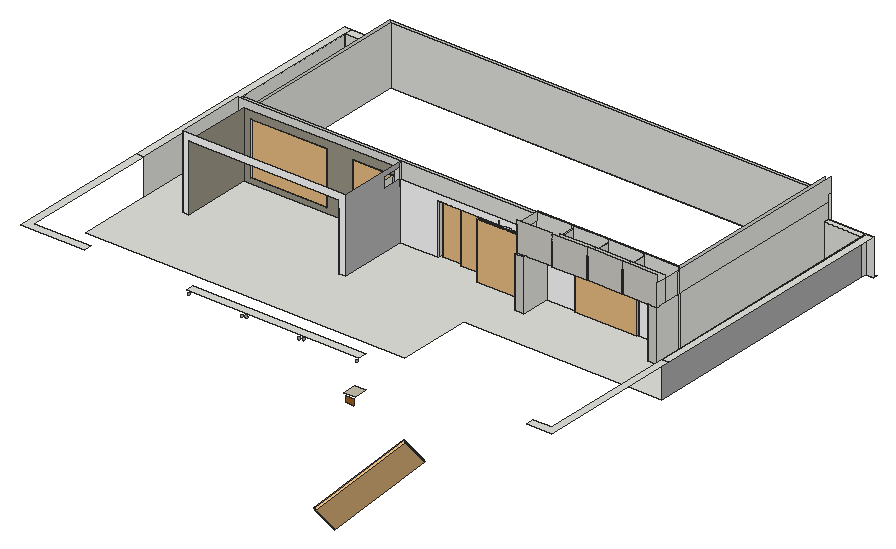
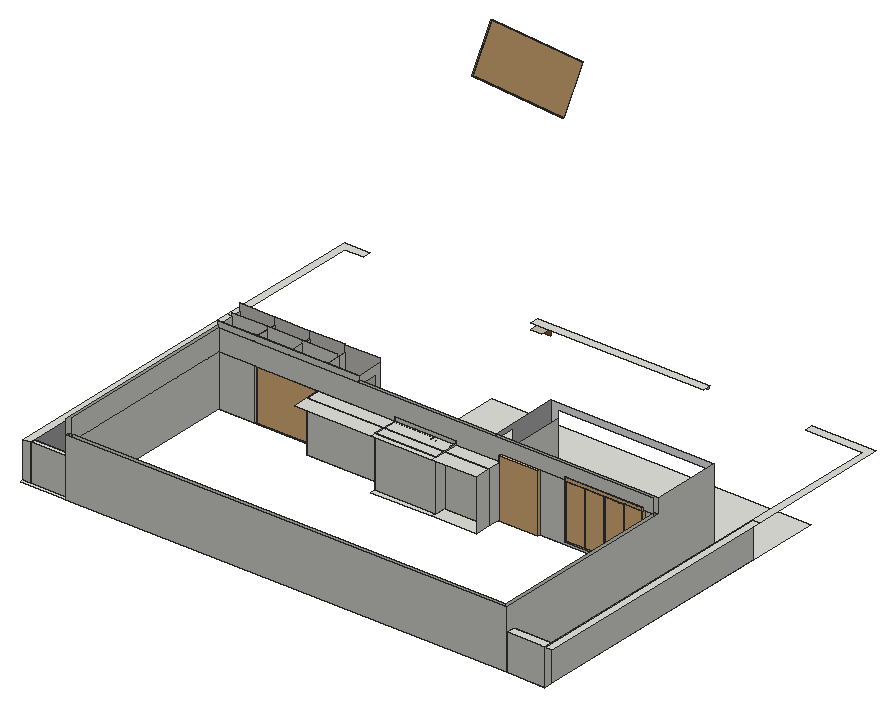
# SketchUp Ruby script. Lengths in inches.
U = 1.inch
M = Sketchup.active_model
def pt(a) = Geom::Point3d.new(a.map { |v| v * U })
def face(e, loops, mat)
  f = e.add_face(loops[0].map { |a| pt(a) })
  loops[1..].each { |l| e.add_face(l.map { |a| pt(a) }).erase! }
  f.material = f.back_material = mat if mat
  f
end
# faces: each face lists its corners as indices into pts; further lists are holes
def faces(e, pts, list, mat = nil) = list.each { |f| face(e, (f[0].is_a?(Array) ? f : [f]).map { |l| l.map { |i| pts[i] } }, mat) }
# xy, xz, yz: faces in a plane at the given z, y or x. An outline is a flat list of corners, or four numbers for a rectangle; further outlines are holes
def ring(l) = l.size == 4 ? [[l[0], l[1]], [l[2], l[1]], [l[2], l[3]], [l[0], l[3]]] : l.each_slice(2).to_a
def flat(e, list, mat, &to3) = list.each { |f| face(e, (f[0].is_a?(Array) ? f : [f]).map { |l| ring(l).map { |u, v| to3.(u, v) } }, mat) }
def xy(e, z, list, mat = nil) = flat(e, list, mat) { |x, y| [x, y, z] }
def xz(e, y, list, mat = nil) = flat(e, list, mat) { |x, z| [x, y, z] }
def yz(e, x, list, mat = nil) = flat(e, list, mat) { |y, z| [x, y, z] }
def lines(e, pts, list) = list.each { |a, b| e.add_line(pt(pts[a]), pt(pts[b])) }
# prism: a flat outline (further loops are holes) pulled along v
def prism(e, loops, v, mat = nil)
  f = face(e, loops, mat); d = Geom::Vector3d.new(v.map { |x| x * U })
  f.pushpull(f.normal.samedirection?(d) ? d.length : -d.length)
end
def box(e, o, s, mat = nil) = prism(e, [[o, [o[0] + s[0], o[1], o[2]], [o[0] + s[0], o[1] + s[1], o[2]], [o[0], o[1] + s[1], o[2]]]], [0, 0, s[2]], mat)
def at(x, y, z, deg = 0) = Geom::Transformation.translation(pt([x, y, z])) * Geom::Transformation.rotation(ORIGIN, Z_AXIS, deg.degrees)
def axes(o, x, y, z) = Geom::Transformation.new([*x, 0, *y, 0, *z, 0, *pt(o).to_a, 1])
def part(name) = M.definitions.add(name)
# library, detail: a bought-in or finely detailed component or shape, given as its bounding box
def library(name, o, s) = part(name).tap { |d| box(d.entities, o, s) }
def detail(e, o, s) = box(e.add_group.entities, o, s)
def put(e, d, t, mat = nil) = e.add_instance(d, t).tap { |i| i.material = mat if mat }
def group(e, t, mat = nil) = e.add_group.tap { |g| g.transformation = t; g.material = mat if mat }.entities
root = M.entities
M.materials.add("Material~3").color = [123, 113, 102]
M.materials.add("[0128_White]").color = [255, 255, 255]
M.materials.add("[0129_WhiteSmoke]").color = [178, 178, 178]
M.materials.add("[0132_LightGray]").color = [169, 169, 169]
M.materials.add("[Concrete Tile]").color = [155, 150, 134]
M.materials.add("[Terrazzo Tile Light]").color = [209, 207, 200]
M.materials.add("[Tile Canvas]").color = [199, 192, 173]
M.materials.add("[Wood Square Tile 02]").color = [160, 95, 34]
c1 = library("3DGeom~4_Defintion",[362.52,-15.59,12.6],[288.85,70.11,1000])
c2 = library("3 door",[0,0,0],[74.8,3.9375,43.31])
c3 = library("door (1)",[38.93,25.48,0],[40,9.94,82.68])
c4 = library("JALI+PATTERN-03",[8.875,53.125,6.4375],[84,1,53.5])
c5 = library("Group\#167",[0,0,0],[77.52,5,145.33])
xy(root,5.1875,[[[2048.43,611.53,2576.35,611.53,2576.35,732.28,2904.07,732.28,2904.07,1146.63,2840.8125,1146.63,2840.8125,851.0625,2671.4,851.0625,2671.4,845.35,2623.94,845.35,2623.94,798.41,2608.61,798.41,2608.61,845.35,2544.33,845.35,2544.33,874.25,2444.05,874.25,2444.05,845.35,2381.36,845.35,2381.36,732.28,2370.42,732.28,2370.42,851.0625,2305.05,851.0625,2305.05,845.35,2123,845.35,2123,732.28,2112.0625,732.28,2112.0625,1146.63,2048.43,1146.63],[2825.48,801.78,2840.8125,845.35]],[2112.0625,732.28,2112.0625,1160.85,2916.0625,1160.85,2916.0625,1155.13,2117.78,1155.13,2117.78,851.0625,2305.05,851.0625,2305.05,845.35,2123,845.35,2123,732.28],[2370.42,732.28,2370.42,846.1,2444.05,846.1,2444.05,845.35,2381.36,845.35,2381.36,732.28],[2608.61,798.41,2608.61,845.35,2544.33,845.35,2544.33,846.1,2671.4,846.1,2671.4,845.35,2623.94,845.35,2623.94,798.41],[2825.48,801.78,2840.8125,845.35],
  [2370.42,846.1,2444.05,874.25],[2544.33,846.1,2671.4,874.25],[2835.1,851.0625,2840.8125,1155.13],[2370.42,874.25,2444.05,900.375],[2444.05,874.25,2544.33,892.35],
  [2444.05,892.35,2544.33,900.375],[2048.43,1146.63,2112.0625,1160.85],[2840.8125,1146.63,2904.07,1155.13]])
xy(root,13.84,[[2134.72,845.35,2259.6,851.0625]])
xy(root,32.74,[[2602.58,453.42,2621.02,475.99]],"[Tile Canvas]")
xy(root,65.1875,[[2036.8125,491.47,2142.71,491.47,2142.71,505.1,2048.43,505.1,2048.43,732.28,2036.8125,732.28],[2311.71,491.47,2596.56,505.1],[2873.37,491.47,2916.0625,491.47,2916.0625,732.28,2904.07,732.28,2904.07,505.1,2873.37,505.1],[2036.8125,732.28,2048.43,1160.85],[2904.07,732.28,2916.0625,1155.13],
  [2048.43,1146.63,2112.0625,1160.85],[2840.8125,1146.63,2904.07,1155.13]])
xy(root,89.42,[[2608.61,798.41,2623.94,801.78],[2623.94,801.78,2666.66,814.22],[2667.6,801.78,2671.4,817.6],[2671.4,801.78,2724.71,817.6],[2725.77,801.78,2776.01,817.6],
  [2776.01,801.78,2782.76,817.6],[2784.08,801.78,2825.48,817.6],[2825.48,801.78,2840.8125,817.6],[2623.94,814.22,2666.66,844.47],[2667.6,817.6,2671.4,844.47],
  [2671.4,817.6,2724.71,844.47],[2725.77,817.6,2776.01,844.47],[2776.01,817.6,2782.76,844.47],[2784.08,817.6,2825.48,844.47],[2825.48,817.6,2840.8125,844.47],
  [2608.61,844.47,2623.94,845.35],[2623.94,844.47,2671.4,845.35],[2671.4,844.47,2776.01,845.35],[2776.01,844.47,2825.48,845.35],[2825.48,844.47,2840.8125,845.35],
  [2444.05,845.35,2544.33,846.1],[2544.33,845.35,2608.61,846.1],[2608.61,845.35,2671.4,846.1],[2671.4,845.35,2776.01,846.1],[2776.01,845.35,2840.8125,846.1],
  [2370.42,846.1,2444.05,851.0625],[2544.33,846.1,2671.4,851.0625],[2671.4,846.1,2776.01,851.0625],[2776.01,846.1,2840.8125,851.0625],[2370.42,851.0625,2444.05,874.25],
  [2444.05,851.0625,2544.33,874.25],[2544.33,851.0625,2671.4,874.25],[2835.1,851.0625,2840.8125,1155.13],[2370.42,874.25,2444.05,900.375],[2444.05,874.25,2544.33,892.35],
  [2544.33,874.25,2671.4,900.375],[2444.05,892.35,2544.33,900.375]])
xz(root,453.42,[[2604.93,19.53,2619.05,29.34]],"[Wood Square Tile 02]")
xz(root,491.47,[[2402.92,57.74,2403.41,57.8,2403.86,57.99,2404.25,58.29,2404.55,58.68,2404.73,59.13,2404.8,59.61,2404.73,60.1,2404.55,60.55,2404.25,60.94,2403.86,61.24,2403.41,61.43,2402.92,61.49,2402.4375,61.43,2401.99,61.24,2401.6,60.94,2401.3,60.55,2401.11,60.1,2401.05,59.61,2401.11,59.13,2401.3,58.68,2401.6,58.29,2401.99,57.99,2402.4375,57.8],[2497.875,57.74,2498.36,57.8,2498.8125,57.99,2499.2,58.29,2499.5,58.68,2499.69,59.13,2499.75,59.61,2499.69,60.1,2499.5,60.55,2499.2,60.94,2498.8125,61.24,2498.36,61.43,2497.875,61.49,2497.39,61.43,2496.9375,61.24,2496.55,60.94,2496.25,60.55,2496.0625,60.1,2496,59.61,2496.0625,59.13,2496.25,58.68,2496.55,58.29,2496.9375,57.99,2497.39,57.8],[2592.82,57.74,2593.31,57.8,2593.76,57.99,2594.15,58.29,2594.45,58.68,2594.64,59.13,2594.7,59.61,2594.64,60.1,2594.45,60.55,2594.15,60.94,2593.76,61.24,2593.31,61.43,2592.82,61.49,2592.34,61.43,2591.89,61.24,2591.5,60.94,2591.2,60.55,2591.01,60.1,2590.95,59.61,2591.01,59.13,2591.2,58.68,2591.5,58.29,2591.89,57.99,2592.34,57.8],[2315.19,59.21,2315.68,59.22,2316.15,59.36,2316.57,59.61,2316.9,59.97,2317.14,60.4,2317.25,60.875,2317.24,61.36,2317.1,61.83,2316.85,62.25,2316.49,62.59,2316.07,62.82,2315.59,62.9375,2315.1,62.93,2314.63,62.79,2314.21,62.53,2313.875,62.18,2313.64,61.75,2313.53,61.27,2313.54,60.78,2313.68,60.32,2313.93,59.9,2314.28,59.56,2314.71,59.33],[2410.14,59.21,2410.63,59.22,2411.1,59.36,2411.52,59.61,2411.86,59.97,2412.09,60.4,2412.2,60.875,2412.19,61.36,2412.05,61.83,2411.8,62.25,2411.45,62.59,2411.02,62.82,2410.54,62.9375,2410.05,62.93,2409.58,62.79,2409.16,62.53,2408.83,62.18,2408.59,61.75,2408.48,61.27,2408.49,60.78,2408.625,60.32,2408.88,59.9,2409.24,59.56,2409.67,59.33],
  [2505.09,59.21,2505.58,59.22,2506.05,59.36,2506.47,59.61,2506.81,59.97,2507.04,60.4,2507.16,60.875,2507.14,61.36,2507.01,61.83,2506.75,62.25,2506.4,62.59,2505.97,62.82,2505.49,62.9375,2505,62.93,2504.53,62.79,2504.11,62.53,2503.78,62.18,2503.54,61.75,2503.43,61.27,2503.4375,60.78,2503.58,60.32,2503.83,59.9,2504.1875,59.56,2504.62,59.33]],"[0132_LightGray]")
xz(root,732.28,[[2112.0625,5.1875,2123,5.1875,2123,114.25,2370.42,114.25,2370.42,5.1875,2381.36,5.1875,2381.36,125.1875,2112.0625,125.1875]],"[0128_White]")
xz(root,798.41,[[2608.61,5.1875,2623.94,89.42]],"[Terrazzo Tile Light]")
xz(root,801.78,[[2825.48,5.1875,2840.8125,89.42],[[2608.61,89.42,2666.66,138.0625],[2612.5,131.88,2612.21,131.92,2611.93,132.03,2611.7,132.21,2611.52,132.44,2611.41,132.71,2611.37,133,2611.41,133.29,2611.52,133.57,2611.7,133.8,2611.93,133.98,2612.21,134.09,2612.5,134.13,2612.79,134.09,2613.06,133.98,2613.29,133.8,2613.47,133.57,2613.58,133.29,2613.62,133,2613.58,132.71,2613.47,132.44,2613.29,132.21,2613.06,132.03,2612.79,131.92],[2663.62,131.88,2663.33,131.92,2663.06,132.03,2662.83,132.21,2662.65,132.44,2662.53,132.71,2662.5,133,2662.53,133.29,2662.65,133.57,2662.83,133.8,2663.06,133.98,2663.33,134.09,2663.62,134.13,2663.91,134.09,2664.18,133.98,2664.42,133.8,2664.6,133.57,2664.71,133.29,2664.75,133,2664.71,132.71,2664.6,132.44,2664.42,132.21,2664.18,132.03,2663.91,131.92],[2663.62,91.63,2663.33,91.67,2663.06,91.78,2662.83,91.96,2662.65,92.19,2662.53,92.46,2662.5,92.75,2662.53,93.04,2662.65,93.32,2662.83,93.55,2663.06,93.73,2663.33,93.84,2663.62,93.88,2663.91,93.84,2664.18,93.73,2664.42,93.55,2664.6,93.32,2664.71,93.04,2664.75,92.75,2664.71,92.46,2664.6,92.19,2664.42,91.96,2664.18,91.78,2663.91,91.67],[2611.43,91.63,2611.14,91.67,2610.87,91.78,2610.64,91.96,2610.46,92.19,2610.35,92.46,2610.31,92.75,2610.35,93.04,2610.46,93.32,2610.64,93.55,2610.87,93.73,2611.14,93.84,2611.43,93.88,2611.73,93.84,2612,93.73,2612.23,93.55,2612.41,93.32,2612.52,93.04,2612.56,92.75,2612.52,92.46,2612.41,92.19,2612.23,91.96,2612,91.78,2611.73,91.67]],[[2667.6,89.42,2724.71,138.0625],[2671.48,131.88,2671.19,131.92,2670.92,132.03,2670.6875,132.21,2670.51,132.44,2670.4,132.71,2670.36,133,2670.4,133.29,2670.51,133.57,2670.6875,133.8,2670.92,133.98,2671.19,134.09,2671.48,134.13,2671.78,134.09,2672.05,133.98,2672.28,133.8,2672.46,133.57,2672.57,133.29,2672.61,133,2672.57,132.71,2672.46,132.44,2672.28,132.21,2672.05,132.03,2671.78,131.92],[2722.61,91.63,2722.32,91.67,2722.05,91.78,2721.8125,91.96,2721.64,92.19,2721.52,92.46,2721.48,92.75,2721.52,93.04,2721.64,93.32,2721.8125,93.55,2722.05,93.73,2722.32,93.84,2722.61,93.88,2722.9,93.84,2723.17,93.73,2723.41,93.55,2723.58,93.32,2723.7,93.04,2723.73,92.75,2723.7,92.46,2723.58,92.19,2723.41,91.96,2723.17,91.78,2722.9,91.67],[2670.42,91.63,2670.13,91.67,2669.86,91.78,2669.625,91.96,2669.45,92.19,2669.34,92.46,2669.3,92.75,2669.34,93.04,2669.45,93.32,2669.625,93.55,2669.86,93.73,2670.13,93.84,2670.42,93.88,2670.71,93.84,2670.98,93.73,2671.22,93.55,2671.4,93.32,2671.51,93.04,2671.55,92.75,2671.51,92.46,2671.4,92.19,2671.22,91.96,2670.98,91.78,2670.71,91.67],[2722.61,131.88,2722.32,131.92,2722.05,132.03,2721.8125,132.21,2721.64,132.44,2721.52,132.71,2721.48,133,2721.52,133.29,2721.64,133.57,2721.8125,133.8,2722.05,133.98,2722.32,134.09,2722.61,134.13,2722.9,134.09,2723.17,133.98,2723.41,133.8,2723.58,133.57,2723.7,133.29,2723.73,133,2723.7,132.71,2723.58,132.44,2723.41,132.21,2723.17,132.03,2722.9,131.92]],[[2725.77,89.42,2782.76,138.0625],[2780.79,131.88,2780.49,131.92,2780.22,132.03,2779.99,132.21,2779.8125,132.44,2779.7,132.71,2779.66,133,2779.7,133.29,2779.8125,133.57,2779.99,133.8,2780.22,133.98,2780.49,134.09,2780.79,134.13,2781.08,134.09,2781.35,133.98,2781.58,133.8,2781.76,133.57,2781.87,133.29,2781.91,133,2781.87,132.71,2781.76,132.44,2781.58,132.21,2781.35,132.03,2781.08,131.92],[2729.66,131.88,2729.37,131.92,2729.1,132.03,2728.86,132.21,2728.6875,132.44,2728.57,132.71,2728.54,133,2728.57,133.29,2728.6875,133.57,2728.86,133.8,2729.1,133.98,2729.37,134.09,2729.66,134.13,2729.95,134.09,2730.22,133.98,2730.46,133.8,2730.63,133.57,2730.75,133.29,2730.79,133,2730.75,132.71,2730.63,132.44,2730.46,132.21,2730.22,132.03,2729.95,131.92],[2780.79,91.63,2780.49,91.67,2780.22,91.78,2779.99,91.96,2779.8125,92.19,2779.7,92.46,2779.66,92.75,2779.7,93.04,2779.8125,93.32,2779.99,93.55,2780.22,93.73,2780.49,93.84,2780.79,93.88,2781.08,93.84,2781.35,93.73,2781.58,93.55,2781.76,93.32,2781.87,93.04,2781.91,92.75,2781.87,92.46,2781.76,92.19,2781.58,91.96,2781.35,91.78,2781.08,91.67],[2728.6,91.63,2728.31,91.67,2728.04,91.78,2727.8,91.96,2727.625,92.19,2727.51,92.46,2727.47,92.75,2727.51,93.04,2727.625,93.32,2727.8,93.55,2728.04,93.73,2728.31,93.84,2728.6,93.88,2728.89,93.84,2729.16,93.73,2729.39,93.55,2729.57,93.32,2729.68,93.04,2729.72,92.75,2729.68,92.46,2729.57,92.19,2729.39,91.96,2729.16,91.78,2728.89,91.67]],[[2784.08,89.42,2840.8125,138.0625],[2786.9,91.63,2786.61,91.67,2786.34,91.78,2786.1,91.96,2785.92,92.19,2785.8125,92.46,2785.77,92.75,2785.8125,93.04,2785.92,93.32,2786.1,93.55,2786.34,93.73,2786.61,93.84,2786.9,93.88,2787.19,93.84,2787.46,93.73,2787.69,93.55,2787.87,93.32,2787.99,93.04,2788.02,92.75,2787.99,92.46,2787.87,92.19,2787.69,91.96,2787.46,91.78,2787.19,91.67],[2787.96,131.88,2787.67,131.92,2787.4,132.03,2787.17,132.21,2786.99,132.44,2786.875,132.71,2786.84,133,2786.875,133.29,2786.99,133.57,2787.17,133.8,2787.4,133.98,2787.67,134.09,2787.96,134.13,2788.25,134.09,2788.52,133.98,2788.76,133.8,2788.94,133.57,2789.05,133.29,2789.09,133,2789.05,132.71,2788.94,132.44,2788.76,132.21,2788.52,132.03,2788.25,131.92],[2839.09,91.63,2838.8,91.67,2838.52,91.78,2838.29,91.96,2838.11,92.19,2838,92.46,2837.96,92.75,2838,93.04,2838.11,93.32,2838.29,93.55,2838.52,93.73,2838.8,93.84,2839.09,93.88,2839.38,93.84,2839.65,93.73,2839.88,93.55,2840.06,93.32,2840.17,93.04,2840.21,92.75,2840.17,92.46,2840.06,92.19,2839.88,91.96,2839.65,91.78,2839.38,91.67],[2839.09,131.88,2838.8,131.92,2838.52,132.03,2838.29,132.21,2838.11,132.44,2838,132.71,2837.96,133,2838,133.29,2838.11,133.57,2838.29,133.8,2838.52,133.98,2838.8,134.09,2839.09,134.13,2839.38,134.09,2839.65,133.98,2839.88,133.8,2840.06,133.57,2840.17,133.29,2840.21,133,2840.17,132.71,2840.06,132.44,2839.88,132.21,2839.65,132.03,2839.38,131.92]]],"[Terrazzo Tile Light]")
xz(root,817.6,[[2667.6,89.42,2724.71,131.1875],[2725.77,89.42,2782.76,131.1875],[2784.08,89.42,2840.8125,131.1875]])
xz(root,844.47,[[2608.61,89.42,2666.66,131.1875],[2666.66,89.42,2667.6,131.1875],[2667.6,89.42,2724.71,131.1875],[2724.71,89.42,2725.77,131.1875],[2725.77,89.42,2782.76,131.1875],
  [2782.76,89.42,2784.08,131.1875],[2784.08,89.42,2840.8125,131.1875]])
xz(root,845.35,[[2544.33,5.1875,2608.61,89.42],[2825.48,5.1875,2840.8125,89.42]])
xz(root,845.35,[[2381.36,5.1875,2444.05,5.1875,2444.05,89.42,2608.61,89.42,2608.61,99.26,2381.36,99.26],[2623.94,5.1875,2671.4,89.42],[2776.01,5.1875,2825.48,89.42]],"[0128_White]")
xz(root,845.35,[[[2123,5.1875,2305.05,5.1875,2305.05,101.375,2370.42,101.375,2370.42,114.25,2123,114.25],[2134.72,13.84,2259.6,101.78]]],"[Concrete Tile]")
xz(root,846.1,[[2370.42,5.1875,2444.05,89.42],[2544.33,5.1875,2671.4,89.42],[2370.42,89.42,2381.36,89.42,2381.36,125.1875,2112.0625,125.1875,2112.0625,101.375,2370.42,101.375],[2381.36,89.42,2381.36,125.1875,2608.61,125.1875,2608.61,89.42,2544.33,89.42,2544.33,95.79,2444.05,95.79,2444.05,89.42],[2444.05,89.42,2544.33,95.79],
  [2608.61,89.42,2840.8125,131.1875]])
xz(root,851.0625,[[2117.78,5.1875,2117.78,101.375,2134.72,101.375,2134.72,13.84,2259.6,13.84,2259.6,101.375,2305.05,101.375,2305.05,5.1875],[2776.01,5.1875,2835.1,89.42],[2835.1,5.1875,2840.8125,89.42],[2370.42,89.42,2370.42,101.375,2259.6,101.375,2259.6,101.78,2134.72,101.78,2134.72,101.375,2117.78,101.375,2117.78,125.1875,2835.1,125.1875,2835.1,89.42,2544.33,89.42,2544.33,95.79,2444.05,95.79,2444.05,89.42],[2444.05,89.42,2544.33,95.79]])
xz(root,874.25,[[2370.42,5.1875,2671.4,89.42]])
xz(root,892.35,[[2444.05,5.1875,2544.33,89.42]])
xz(root,1146.63,[[2048.43,5.1875,2112.0625,65.1875],[2840.8125,5.1875,2904.07,65.1875]])
xz(root,1155.13,[[2117.78,5.1875,2835.1,101.375],[2835.1,5.1875,2840.8125,89.42],[2840.8125,5.1875,2904.07,65.1875],[2904.07,5.1875,2916.0625,65.1875],[2835.1,89.42,2840.8125,101.375]])
xz(root,1160.85,[[2048.43,5.1875,2112.0625,65.1875],[2112.0625,5.1875,2840.8125,101.375]])
yz(root,2048.43,[[732.28,5.1875,1146.63,65.1875],[1146.63,5.1875,1160.85,65.1875]])
yz(root,2112.0625,[[732.28,5.1875,732.28,125.1875,846.1,125.1875,846.1,101.375,1160.85,101.375,1160.85,65.1875,1146.63,65.1875,1146.63,5.1875],[1146.63,5.1875,1160.85,65.1875]])
yz(root,2117.78,[[851.0625,5.1875,1155.13,101.375]])
yz(root,2123,[[732.28,5.1875,845.35,114.25]],"[Concrete Tile]")
yz(root,2134.72,[[845.35,13.84,851.0625,101.78]])
yz(root,2259.6,[[845.35,13.84,851.0625,101.78]])
yz(root,2305.05,[[845.35,5.1875,851.0625,101.375]])
yz(root,2370.42,[[732.28,5.1875,846.1,101.375],[846.1,5.1875,874.25,89.42],[874.25,5.1875,900.375,89.42],[846.1,89.42,851.0625,101.375]])
yz(root,2381.36,[[845.35,89.42,846.1,125.1875]])
yz(root,2381.36,[[732.28,5.1875,845.35,5.1875,845.35,99.26,810.97,99.26,810.97,117.26,845.35,117.26,845.35,125.1875,732.28,125.1875]],"[0129_WhiteSmoke]")
yz(root,2444.05,[[845.35,5.1875,846.1,89.42],[846.1,5.1875,892.35,89.42],[846.1,89.42,851.0625,95.79]])
yz(root,2544.33,[[845.35,5.1875,846.1,89.42],[846.1,5.1875,892.35,89.42],[846.1,89.42,851.0625,95.79]])
yz(root,2608.61,[[798.41,5.1875,798.41,89.42,801.78,89.42,801.78,131.1875,844.47,131.1875,844.47,117.26,810.97,117.26,810.97,99.26,844.47,99.26,844.47,89.42,845.35,89.42,845.35,5.1875],[844.47,89.42,845.35,99.26],[845.35,89.42,846.1,125.1875]])
yz(root,2623.94,[[798.41,5.1875,845.35,89.42]])
yz(root,2666.66,[[801.78,89.42,814.22,125.1875],[814.22,89.42,844.47,125.1875]])
yz(root,2667.6,[[801.78,89.42,817.6,125.1875],[817.6,89.42,844.47,125.1875]])
yz(root,2671.4,[[845.35,5.1875,846.1,89.42],[846.1,5.1875,874.25,89.42]])
yz(root,2724.71,[[801.78,89.42,817.6,125.1875],[817.6,89.42,844.47,125.1875]])
yz(root,2725.77,[[801.78,89.42,817.6,125.1875],[817.6,89.42,844.47,125.1875]])
yz(root,2776.01,[[845.35,5.1875,851.0625,89.42]])
yz(root,2782.76,[[801.78,89.42,817.6,125.1875],[817.6,89.42,844.47,125.1875]])
yz(root,2784.08,[[801.78,89.42,817.6,125.1875],[817.6,89.42,844.47,125.1875]])
yz(root,2825.48,[[801.78,5.1875,845.35,89.42]])
yz(root,2835.1,[[851.0625,5.1875,1155.13,89.42],[851.0625,89.42,1155.13,125.1875]])
yz(root,2840.8125,[[801.78,5.1875,845.35,89.42],[851.0625,5.1875,1146.63,5.1875,1146.63,65.1875,1155.13,65.1875,1155.13,89.42,851.0625,89.42],[1146.63,5.1875,1155.13,65.1875],[801.78,89.42,817.6,125.1875],[817.6,89.42,844.47,125.1875],
  [844.47,89.42,846.1,125.1875],[846.1,89.42,1155.13,89.42,1155.13,101.375,1160.85,101.375,1160.85,125.1875,846.1,125.1875]])
yz(root,2904.07,[[1146.63,5.1875,1155.13,65.1875]])
yz(root,2904.07,[[732.28,5.1875,1146.63,65.1875]],"[0132_LightGray]")
p = [[2608.61,814.22,89.42],[2623.94,814.22,89.42]]
lines(root,p,[[0,1]])
put(root,c1,axes([2092.12,853.3125,12.94],[0.11056,0,0],[0,-0.05859,0],[0,0,0.08734]),"Material~3")
put(root,c1,axes([2123.59,853.99,12.94],[0.11056,0,0],[0,-0.05859,0],[0,0,0.08734]),"Material~3")
put(root,c2,axes([2134.72,847.72,10.15],[1.71563,0,0],[0,1.38,0],[0,0,2.21476]))
put(root,c1,axes([2155.65,853.99,12.94],[0.11056,0,0],[0,-0.05859,0],[0,0,0.08734]),"Material~3")
put(root,c1,axes([2187.72,853.99,12.94],[0.11056,0,0],[0,-0.05859,0],[0,0,0.08734]),"Material~3")
put(root,c3,axes([2241.42,814.19,5.1875],[1.63437,0,0],[0,1.16,0],[0,0,1.16]))
put(root,c1,axes([2407,857.09,3.96],[0.11056,0,0],[0,-0.11056,0],[0,0,0.08439]),"Material~3")
put(root,c1,axes([2440.38,851.7,3.96],[0.11056,0,0],[0,-0.08955,0],[0,0,0.08439]),"Material~3")
put(root,c1,axes([2472.32,851.7,3.96],[0.11056,0,0],[0,-0.08955,0],[0,0,0.08439]),"Material~3")
put(root,c4,axes([2513.96,766.91,109.2],[0,0,-1.12],[0,1.12,0],[1.5792,0,0]))
put(root,c2,axes([2671.4,843.85,5.1875],[1.38,0,0],[0,1.38,0],[0,0,1.94496]))
put(root,c5,axes([2874.64,90.72,88.69],[0.1418,-0.68301,0.71651],[0.87033,-0.25882,-0.41896],[0.4716,0.68301,0.55775]))
